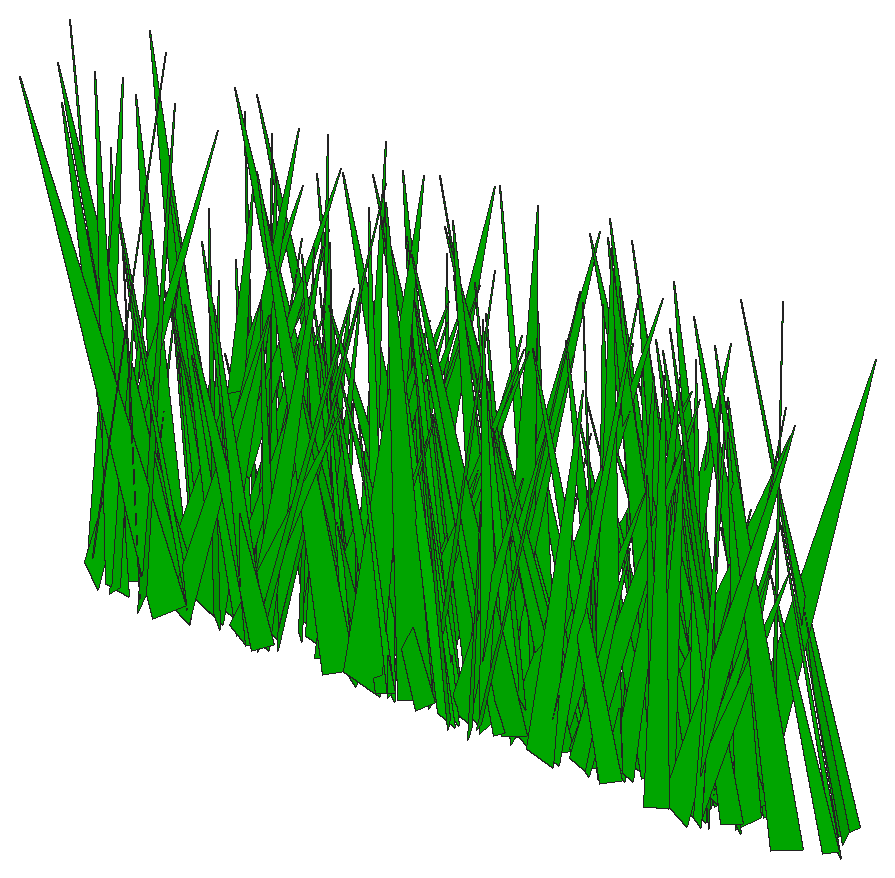
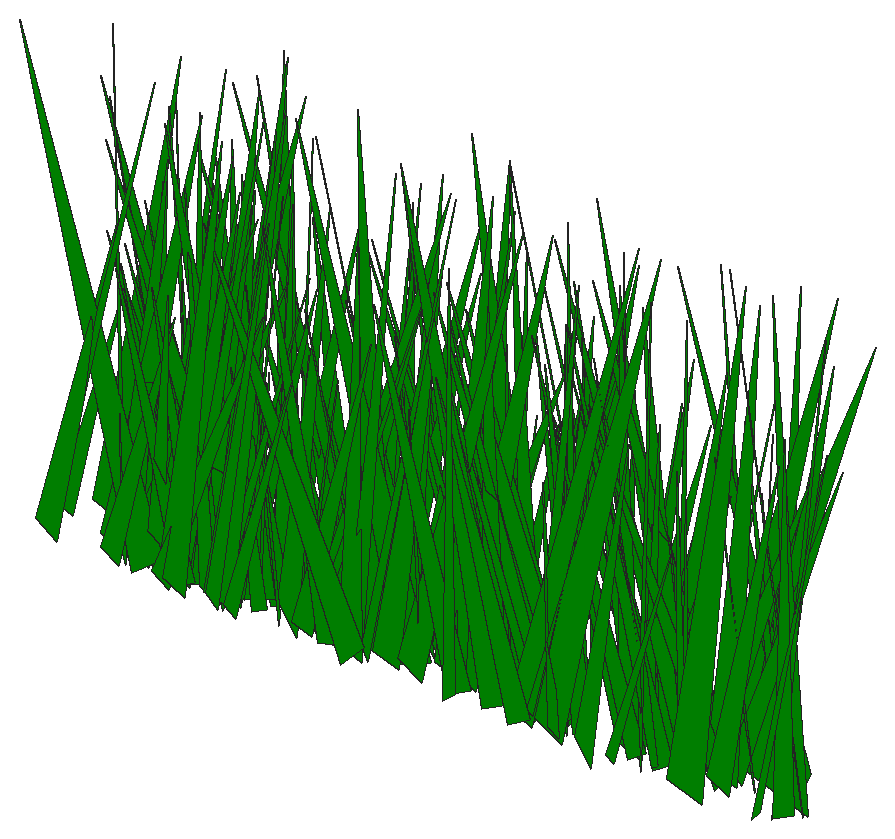
# SketchUp Ruby script. Lengths in inches.
U = 1.inch
M = Sketchup.active_model
def pt(a) = Geom::Point3d.new(a.map { |v| v * U })
def face(e, loops, mat)
  f = e.add_face(loops[0].map { |a| pt(a) })
  loops[1..].each { |l| e.add_face(l.map { |a| pt(a) }).erase! }
  f.material = f.back_material = mat if mat
  f
end
# faces: each face lists its corners as indices into pts; further lists are holes
def faces(e, pts, list, mat = nil) = list.each { |f| face(e, (f[0].is_a?(Array) ? f : [f]).map { |l| l.map { |i| pts[i] } }, mat) }
# xy, xz, yz: faces in a plane at the given z, y or x. An outline is a flat list of corners, or four numbers for a rectangle; further outlines are holes
def ring(l) = l.size == 4 ? [[l[0], l[1]], [l[2], l[1]], [l[2], l[3]], [l[0], l[3]]] : l.each_slice(2).to_a
def flat(e, list, mat, &to3) = list.each { |f| face(e, (f[0].is_a?(Array) ? f : [f]).map { |l| ring(l).map { |u, v| to3.(u, v) } }, mat) }
def xy(e, z, list, mat = nil) = flat(e, list, mat) { |x, y| [x, y, z] }
def xz(e, y, list, mat = nil) = flat(e, list, mat) { |x, z| [x, y, z] }
def yz(e, x, list, mat = nil) = flat(e, list, mat) { |y, z| [x, y, z] }
def lines(e, pts, list) = list.each { |a, b| e.add_line(pt(pts[a]), pt(pts[b])) }
# prism: a flat outline (further loops are holes) pulled along v
def prism(e, loops, v, mat = nil)
  f = face(e, loops, mat); d = Geom::Vector3d.new(v.map { |x| x * U })
  f.pushpull(f.normal.samedirection?(d) ? d.length : -d.length)
end
def box(e, o, s, mat = nil) = prism(e, [[o, [o[0] + s[0], o[1], o[2]], [o[0] + s[0], o[1] + s[1], o[2]], [o[0], o[1] + s[1], o[2]]]], [0, 0, s[2]], mat)
def at(x, y, z, deg = 0) = Geom::Transformation.translation(pt([x, y, z])) * Geom::Transformation.rotation(ORIGIN, Z_AXIS, deg.degrees)
def axes(o, x, y, z) = Geom::Transformation.new([*x, 0, *y, 0, *z, 0, *pt(o).to_a, 1])
def part(name) = M.definitions.add(name)
# library, detail: a bought-in or finely detailed component or shape, given as its bounding box
def library(name, o, s) = part(name).tap { |d| box(d.entities, o, s) }
def detail(e, o, s) = box(e.add_group.entities, o, s)
def put(e, d, t, mat = nil) = e.add_instance(d, t).tap { |i| i.material = mat if mat }
def group(e, t, mat = nil) = e.add_group.tap { |g| g.transformation = t; g.material = mat if mat }.entities
root = M.entities
M.materials.add("[Color G06]").color = [0, 204, 0]
c1 = part("fur_instance\#9")
p = [[0.8125,0,1.79],[0.67,-0.02,1.48],[0,-0.11,0],[0,0.11,0]]
faces(c1.entities,p,[[0,1,2,3]])
put(root,c1,axes([35.12,20.5,4.28],[3.03106,0.62127,0.65652],[4.35449,-0.39194,-2.30003],[1.03981,-0.16965,7.71826]),"[Color G06]")
put(root,c1,axes([19.64,20.68,4.28],[-0.16092,-0.52107,1.62952],[-3.59911,-0.03804,-2.19139],[-1.48269,0.1489,5.14257]),"[Color G06]")
put(root,c1,axes([19.41,20.69,4.28],[0.64346,-0.50098,1.74087],[-3.60806,-0.13024,-1.32649],[-1.11623,0.13218,5.29122]),"[Color G06]")
put(root,c1,axes([35.98,20.48,4.28],[-4.26408,0.16313,3.37539],[0.76507,0.66856,-1.55286],[2.42564,0.0759,6.42343]),"[Color G06]")
put(root,c1,axes([16.83,20.84,4.28],[-4.57704,-0.06266,0.97472],[-0.21793,0.61243,2.2369],[0.76142,-0.20138,6.49945]),"[Color G06]")
put(root,c1,axes([19.34,20.78,4.28],[4.92761,0.10985,0.51711],[0.85255,-0.66121,-2.01124],[-0.11605,-0.19308,7.18189]),"[Color G06]")
put(root,c1,axes([34.49,20.44,4.28],[2.21235,0.64995,0.69926],[4.55515,-0.31532,1.47593],[-1.0927,0.00144,7.56847]),"[Color G06]")
put(root,c1,axes([35.93,21.02,4.28],[-4.71268,-0.24632,3.19454],[-0.77772,0.68157,3.47433],[2.6616,-0.23699,6.67152]),"[Color G06]")
put(root,c1,axes([26.68,20.53,4.28],[-4.24437,-0.06717,1.88959],[-0.90731,0.57193,-2.21683],[1.00363,0.23297,5.987]),"[Color G06]")
put(root,c1,axes([25.04,21.02,4.28],[1.87576,-0.80358,0.85838],[-5.66872,-0.272,-1.58046],[-1.18508,0.02914,8.91863]),"[Color G06]")
put(root,c1,axes([39.03,20.82,4.28],[0.00921,-0.7447,2.68248],[-5.44964,-0.06467,-2.02075],[-1.42936,0.24178,7.72166]),"[Color G06]")
put(root,c1,axes([27.5,20.5,4.28],[2.69023,0.2021,0.81048],[0.96941,-0.33831,2.5036],[-1.2062,0.17886,3.81975]),"[Color G06]")
put(root,c1,axes([19.36,20.75,4.28],[-2.87953,-0.43874,1.8429],[-3.37542,0.38429,-1.27127],[0.16259,0.20765,6.24647]),"[Color G06]")
put(root,c1,axes([30.03,20.59,4.28],[-0.85297,0.60878,1.16187],[4.29251,0.14106,-1.45105],[1.11278,-0.07747,6.48798]),"[Color G06]")
put(root,c1,axes([24.27,20.86,4.28],[-2.92029,0.05795,1.28824],[0.62873,0.40718,1.07968],[0.72134,-0.12032,4.2743]),"[Color G06]")
put(root,c1,axes([35.49,20.8,4.28],[2.18325,-0.4105,0.47109],[-2.76341,-0.26295,2.28609],[1.06249,0.15961,4.97782]),"[Color G06]")
put(root,c1,axes([15.07,20.6875,4.28],[-3.72344,0.00901,1.8687],[-0.1721,0.53817,-1.06414],[1.24011,0.10175,5.46312]),"[Color G06]")
put(root,c1,axes([16.21,20.62,4.28],[-2.3339,0.80888,0.33748],[5.3635,0.28748,3.69996],[-2.22077,-0.15576,8.58131]),"[Color G06]")
put(root,c1,axes([18.57,20.84,4.28],[2.41753,-0.38371,0.07703],[-2.51991,-0.30476,2.26301],[1.10665,0.14429,4.98474]),"[Color G06]")
put(root,c1,axes([30.38,20.73,4.28],[5.62136,-0.17826,1.62606],[-1.45971,-0.78092,1.43755],[-0.82896,0.16627,8.49527]),"[Color G06]")
put(root,c1,axes([14.17,20.625,4.28],[2.74687,0.29235,0.65447],[1.88385,-0.37704,1.68599],[-1.01892,0.09103,4.88158]),"[Color G06]")
put(root,c1,axes([32.51,20.79,4.28],[-3.33536,0.46956,1.16031],[3.453,0.44692,1.39501],[-0.13635,-0.16822,6.94495]),"[Color G06]")
put(root,c1,axes([35.52,20.76,4.28],[3.05836,-0.22556,0.72653],[-1.67747,-0.38928,1.88997],[0.19704,0.18691,4.8131]),"[Color G06]")
put(root,c1,axes([34.02,21.12,4.28],[-2.60033,-0.46267,0.25722],[-3.10158,0.34898,2.06931],[1.19093,-0.10135,5.9508]),"[Color G06]")
put(root,c1,axes([16.48,20.74,4.28],[2.02147,0.50228,0.40268],[3.50973,-0.26296,-1.67687],[0.8536,-0.10826,5.94115]),"[Color G06]")
put(root,c1,axes([34.1,21.12,4.28],[-0.32855,-0.64108,0.01669],[-4.51737,0.04531,1.27825],[0.85387,-0.00698,6.76896]),"[Color G06]")
put(root,c1,axes([27.64,21.27,4.28],[4.3846,-0.48787,0.56481],[-3.03521,-0.56691,-3.62029],[-1.78067,-0.23498,7.56167]),"[Color G06]")
put(root,c1,axes([14.2,20.71,4.28],[-4.583,0.48117,1.87027],[3.37343,0.66218,-1.10489],[1.44648,-0.01979,8.50251]),"[Color G06]")
put(root,c1,axes([22.67,20.93,4.28],[2.25118,0.34416,0.97871],[2.47695,-0.26475,-2.03182],[0.62042,-0.19181,4.56054]),"[Color G06]")
put(root,c1,axes([36.72,21.24,4.28],[-5.18037,-0.44074,0.71566],[-2.90398,0.70198,2.70695],[1.3364,-0.18308,8.65635]),"[Color G06]")
put(root,c1,axes([15.23,20.54,4.28],[5.5582,0.36566,1.922],[1.96819,-0.75378,3.76014],[-2.15785,0.25435,8.38033]),"[Color G06]")
put(root,c1,axes([17.59,21.1,4.28],[4.26432,0.09876,3.43905],[1.41152,-0.63127,-1.82705],[-1.95037,-0.24093,6.19693]),"[Color G06]")
put(root,c1,axes([26.49,20.67,4.28],[-5.24823,0.34183,0.47936],[2.34477,0.72151,-1.75957],[0.78352,0.13044,8.47659]),"[Color G06]")
put(root,c1,axes([24.1,20.8,4.28],[-0.67427,0.46476,0.38897],[3.23485,0.08136,1.35845],[-0.84375,-0.05948,4.89731]),"[Color G06]")
put(root,c1,axes([34.95,21.02,4.28],[3.93696,0.08139,0.63429],[0.66802,-0.53518,-1.37349],[-0.27293,-0.13593,5.78765]),"[Color G06]")
put(root,c1,axes([36.79,21.06,4.28],[-0.11601,-0.52436,1.11552],[-3.72432,-0.00928,-1.36638],[-0.90927,0.10492,5.45426]),"[Color G06]")
put(root,c1,axes([23.22,20.79,4.28],[-0.49886,0.82731,2.40594],[5.98908,0.11619,-1.81578],[1.38616,-0.20428,8.71119]),"[Color G06]")
put(root,c1,axes([25.5,20.92,4.28],[-0.30634,0.47925,1.93309],[3.28373,-0.04526,2.45133],[-1.64365,-0.17974,4.53704]),"[Color G06]")
put(root,c1,axes([31.09,20.98,4.28],[1.57776,-0.32972,0.79265],[-2.38807,-0.19659,1.22427],[0.41125,0.1234,4.06817]),"[Color G06]")
put(root,c1,axes([37.18,21.34,4.28],[3.35801,-0.57328,0.19361],[-3.78603,-0.43991,-2.9546],[-1.60756,-0.16146,7.3629]),"[Color G06]")
put(root,c1,axes([19.23,20.91,4.28],[2.25077,0.58808,1.62519],[4.34639,-0.29243,-1.29023],[0.27748,-0.1897,7.0271]),"[Color G06]")
put(root,c1,axes([28.6,21.31,4.28],[4.65218,-0.31999,3.02467],[-1.4148,-0.68035,-3.4076],[-2.71291,-0.19393,6.96387]),"[Color G06]")
put(root,c1,axes([15.91,21.14,4.28],[-1.41791,-0.8139,1.79723],[-5.73201,0.13912,-2.86391],[-1.62996,0.21876,8.50796]),"[Color G06]")
put(root,c1,axes([32.02,20.88,4.28],[-4.91073,-0.09175,2.93937],[-1.09973,0.71287,-1.54788],[1.75824,0.18962,7.24145]),"[Color G06]")
put(root,c1,axes([26.59,21.13,4.28],[1.04517,-0.44785,0.3848],[-3.08103,-0.12788,1.59541],[0.94243,0.07859,4.78905]),"[Color G06]")
put(root,c1,axes([25.52,21.18,4.28],[5.42184,-0.07885,1.38292],[-0.3993,-0.75684,-1.4605],[-1.00821,-0.1243,8.01532]),"[Color G06]")
put(root,c1,axes([36.54,21.33,4.28],[-3.5413,-0.41182,0.07637],[-2.82796,0.47593,1.90196],[0.85281,-0.1319,6.62408]),"[Color G06]")
put(root,c1,axes([28.61,21.16,4.28],[-2.8689,-0.64055,0.93156],[-4.58066,0.37601,-1.80997],[-0.71213,0.1619,7.88945]),"[Color G06]")
put(root,c1,axes([19.78,21.1875,4.28],[6.16936,0.07955,0.8439],[0.67537,-0.84425,-1.88696],[-0.43372,-0.18313,9.0656]),"[Color G06]")
put(root,c1,axes([35.68,20.85,4.28],[-4.41516,0.36248,1.9516],[2.30711,0.63792,-1.95194],[1.77187,0.07262,7.40458]),"[Color G06]")
put(root,c1,axes([22.27,20.93,4.28],[-0.35866,0.7597,1.88035],[5.33757,-0.00585,2.54559],[-1.66556,-0.18234,7.75287]),"[Color G06]")
put(root,c1,axes([18.78,20.95,4.28],[-1.105,0.42188,0.11857],[2.93685,0.14663,1.20482],[-0.73109,-0.04864,4.66069]),"[Color G06]")
put(root,c1,axes([31.06,21.12,4.28],[3.73719,0.49583,1.01531],[3.52225,-0.46662,-2.78296],[0.8356,-0.25063,7.18986]),"[Color G06]")
put(root,c1,axes([27.48,20.93,4.28],[5.57106,0.18803,0.56765],[1.26489,-0.76851,1.51381],[-0.60214,0.12531,8.43197]),"[Color G06]")
put(root,c1,axes([31.92,21.33,4.28],[3.69445,-0.67086,2.00041],[-4.7944,-0.54145,-1.08036],[-1.3965,0.0841,9.00119]),"[Color G06]")
put(root,c1,axes([22.82,21.14,4.28],[2.54448,0.33779,0.70213],[2.43032,-0.32681,-1.61237],[0.42666,-0.15291,4.99697]),"[Color G06]")
put(root,c1,axes([26.54,21.26,4.28],[-2.97565,0.01103,1.03454],[0.27155,0.40828,1.24463],[0.6416,-0.12164,4.27124]),"[Color G06]")
put(root,c1,axes([13.81,21.05,4.28],[3.82908,-0.09459,2.02127],[-1.05218,-0.53525,1.57494],[-1.08723,0.18486,5.59449]),"[Color G06]")
put(root,c1,axes([23.23,21.22,4.28],[-3.99076,-0.33553,0.30649],[-2.39896,0.54449,-1.29951],[-0.27685,0.11844,6.84243]),"[Color G06]")
put(root,c1,axes([22.52,21.08,4.28],[-4.08598,0.15524,1.44869],[0.93993,0.58036,-1.22225],[1.13814,0.07801,6.21026]),"[Color G06]")
put(root,c1,axes([13.06,20.93,4.28],[5.98017,-0.1921,1.59286],[-1.71071,-0.74768,3.98827],[-0.32724,0.39808,8.25937]),"[Color G06]")
put(root,c1,axes([28.31,21.19,4.28],[-2.50155,0.55606,1.41368],[4.01936,0.30269,2.21007],[-0.80048,-0.21785,6.67933]),"[Color G06]")
put(root,c1,axes([30.36,21.33,4.28],[-1.19018,-0.46633,1.20952],[-3.31811,0.12397,-1.80256],[-0.91021,0.15783,4.98957]),"[Color G06]")
put(root,c1,axes([28.74,21.23,4.28],[4.54535,0.58511,0.37353],[4.11692,-0.60933,-2.25946],[0.8482,-0.17795,8.96505]),"[Color G06]")
put(root,c1,axes([24.04,21.02,4.28],[-3.86115,0.3343,0.70905],[1.95591,0.49689,-3.12007],[1.46517,0.21766,6.03365]),"[Color G06]")
put(root,c1,axes([29.82,21.36,4.28],[1.90983,-0.43639,1.0195],[-3.01462,-0.20749,2.41207],[1.0822,0.19215,4.91998]),"[Color G06]")
put(root,c1,axes([19.29,21.52,4.28],[-2.70255,-0.39023,1.22922],[-2.68009,0.39392,1.20348],[1.15099,0.00098,5.68854]),"[Color G06]")
put(root,c1,axes([34.15,21.53,4.28],[0.15749,-0.83898,2.44528],[-6.10794,-0.06661,-1.74668],[-1.25267,0.21931,8.8241]),"[Color G06]")
put(root,c1,axes([26.29,21.02,4.28],[-4.98773,0.42535,0.0635],[2.86559,0.65716,-2.89905],[1.04623,0.22784,8.24313]),"[Color G06]")
put(root,c1,axes([17.09,21.39,4.28],[3.61493,0.65317,2.23782],[4.91376,-0.46964,-1.98394],[0.19252,-0.27773,8.61759]),"[Color G06]")
put(root,c1,axes([21.77,21.54,4.28],[0.60564,-0.61854,1.69679],[-4.48522,-0.11225,-1.12457],[-0.92052,0.13998,6.59585]),"[Color G06]")
put(root,c1,axes([32.4375,21.44,4.28],[-0.85714,-0.47006,2.60488],[-3.49577,0.19476,1.46779],[1.47663,0.18821,4.9869]),"[Color G06]")
put(root,c1,axes([21.35,21.26,4.28],[3.67043,0.36059,1.03527],[2.49178,-0.5201,1.07645],[-0.97865,0.02816,6.62356]),"[Color G06]")
put(root,c1,axes([28.75,21.28,4.28],[-3.60971,-0.32931,2.99245],[-2.99666,0.47943,-2.01377],[0.77841,0.31855,6.1244]),"[Color G06]")
put(root,c1,axes([26.88,21.32,4.28],[3.19451,-0.29495,1.75851],[-2.41955,-0.38204,2.45717],[0.06335,0.28178,5.17213]),"[Color G06]")
put(root,c1,axes([33.71,21.32,4.28],[-2.17781,0.39947,0.93712],[2.65887,0.31492,-1.61868],[1.23705,0.0264,5.12894]),"[Color G06]")
put(root,c1,axes([14.27,21.46,4.28],[-1.80547,0.67445,1.82053],[4.92501,0.21252,1.86578],[-0.78831,-0.21696,7.48701]),"[Color G06]")
put(root,c1,axes([32.05,21.29,4.28],[2.70727,0.65205,1.32114],[4.48259,-0.39703,1.99169],[-1.59782,-0.00903,7.82601]),"[Color G06]")
put(root,c1,axes([24.07,21.53,4.28],[4.2436,-0.35839,0.16927],[-2.46631,-0.55809,2.37543],[0.7318,0.19737,7.02409]),"[Color G06]")
put(root,c1,axes([26.62,21.39,4.28],[3.30744,0.24109,0.79704],[1.54588,-0.45707,1.55276],[-0.94012,0.09661,5.35736]),"[Color G06]")
put(root,c1,axes([23.5,21.45,4.28],[2.60414,0.1253,1.1158],[0.66224,-0.36787,1.29287],[-0.96237,0.0859,3.90899]),"[Color G06]")
put(root,c1,axes([40.125,21.51,4.28],[-1.7987,0.35882,0.18815],[2.52485,0.24126,1.06131],[-0.51223,-0.07079,4.57067]),"[Color G06]")
put(root,c1,axes([23.78,21.84,4.28],[5.07038,0.2388,0.6504],[1.69099,-0.60234,-4.04173],[0.5124,-0.37521,6.90232]),"[Color G06]")
put(root,c1,axes([35.47,21.77,4.28],[5.18688,0.03411,1.13883],[0.44504,-0.70208,-2.11198],[-0.66512,-0.20376,7.46789]),"[Color G06]")
put(root,c1,axes([35.07,21.61,4.28],[0.23409,0.45872,2.43222],[3.38187,-0.1153,1.77092],[-1.42577,-0.19816,4.59988]),"[Color G06]")
put(root,c1,axes([15.09,21.63,4.28],[-3.24987,-0.41215,0.45613],[-2.87294,0.41976,-2.15305],[-0.75829,0.17602,6.20239]),"[Color G06]")
put(root,c1,axes([16.12,21.63,4.28],[-1.97766,0.50406,1.12542],[3.46058,0.2115,2.70201],[-1.28752,-0.20578,5.53376]),"[Color G06]")
put(root,c1,axes([27.38,21.78,4.28],[2.40972,-0.65697,2.77663],[-4.71727,-0.39556,-1.60647],[-1.84257,0.1535,7.7441]),"[Color G06]")
put(root,c1,axes([26.76,21.87,4.28],[0.27251,-0.5049,0.06103],[-3.50501,-0.03821,-1.3579],[-0.90901,-0.00401,5.25414]),"[Color G06]")
put(root,c1,axes([17.48,21.7,4.28],[3.79399,-0.27301,0.18763],[-1.93574,-0.51476,1.3933],[0.31881,0.12341,6.22688]),"[Color G06]")
put(root,c1,axes([32.19,21.39,4.28],[-4.10626,0.43516,0.58348],[2.85415,0.55323,-2.53012],[1.32084,0.15737,7.28118]),"[Color G06]")
put(root,c1,axes([30.22,21.74,4.28],[-3.29677,-0.6573,1.53149],[-4.70067,0.39892,-2.93517],[-1.08265,0.26948,8.08042]),"[Color G06]")
put(root,c1,axes([23.38,21.42,4.28],[-4.88738,0.35685,1.49787],[2.1409,0.67312,-2.81805],[1.72335,0.17582,7.74879]),"[Color G06]")
put(root,c1,axes([31.58,21.53,4.28],[-2.66533,0.26974,0.25786],[1.80189,0.35872,-1.50297],[0.72445,0.10019,4.687]),"[Color G06]")
put(root,c1,axes([19.29,21.41,4.28],[5.38754,0.19095,3.5059],[0.36145,-0.77054,3.58038],[-2.69204,0.27869,7.49702]),"[Color G06]")
put(root,c1,axes([32.375,21.96,4.28],[-0.98444,-0.64933,1.24012],[-4.60765,0.15835,1.35416],[1.06832,0.0846,6.98327]),"[Color G06]")
put(root,c1,axes([16.68,21.6,4.28],[-1.52174,0.33683,0.27529],[2.20042,0.20488,-1.62616],[1.01327,0.06095,3.9448]),"[Color G06]")
put(root,c1,axes([25.5625,21.78,4.28],[-0.67103,0.57299,2.52442],[3.89391,-0.03882,3.3244],[-2.13888,-0.25045,5.26021]),"[Color G06]")
put(root,c1,axes([17.5625,21.75,4.28],[-1.88148,0.58726,1.76168],[4.34734,0.2317,1.49858],[-0.47559,-0.20535,6.72902]),"[Color G06]")
put(root,c1,axes([35.65,21.75,4.28],[2.24277,-0.31165,1.59448],[-2.47175,-0.2693,1.71954],[0.15293,0.21775,4.40863]),"[Color G06]")
put(root,c1,axes([33.28,21.77,4.28],[-2.21003,0.46612,0.66655],[3.31705,0.28707,1.50624],[-0.60781,-0.12819,5.79654]),"[Color G06]")
put(root,c1,axes([33.21,21.85,4.28],[1.96878,0.63767,2.01723],[4.34383,-0.15593,-3.80749],[1.96579,-0.29407,6.39314]),"[Color G06]")
put(root,c1,axes([12.36,22.1,4.28],[4.87288,-0.42927,1.62301],[-2.9059,-0.69439,-1.60957],[-1.48722,-0.04974,8.46277]),"[Color G06]")
put(root,c1,axes([15.28,22.02,4.28],[2.16634,-0.67824,2.53769],[-4.87924,-0.35255,-1.51985],[-1.65314,0.15175,7.81131]),"[Color G06]")
put(root,c1,axes([32.36,22.14,4.28],[-0.23066,-0.71514,0.54641],[-4.99104,0.0434,1.81849],[1.23454,0.04184,7.45396]),"[Color G06]")
put(root,c1,axes([40.23,21.6875,4.28],[-3.79499,0.10997,0.12265],[0.71153,0.49705,-2.0156],[0.34977,0.18198,5.43109]),"[Color G06]")
put(root,c1,axes([31.61,22.06,4.28],[1.30861,-0.49054,0.09105],[-3.45578,-0.17751,1.08591],[0.66023,0.04314,5.50344]),"[Color G06]")
put(root,c1,axes([14.41,21.63,4.28],[3.90257,0.21687,0.92757],[1.13038,-0.50313,2.88964],[-1.23536,0.22473,5.5743]),"[Color G06]")
put(root,c1,axes([22.42,21.83,4.28],[4.88543,-0.34726,3.68876],[-3.00301,-0.7191,1.10746],[-1.80971,0.25582,8.12036]),"[Color G06]")
put(root,c1,axes([15.49,21.78,4.28],[3.06956,0.66655,0.29466],[4.64934,-0.40793,-2.18422],[1.12751,-0.13254,8.20453]),"[Color G06]")
put(root,c1,axes([16.82,22.16,4.28],[-0.65445,-0.71745,1.06277],[-5.05125,0.11118,1.67399],[1.20909,0.07615,7.56868]),"[Color G06]")
put(root,c1,axes([33.54,21.9,4.28],[1.06131,0.6918,2.98216],[5.15125,-0.20838,1.45808],[-1.43475,-0.23642,7.44099]),"[Color G06]")
put(root,c1,axes([20.97,22.06,4.28],[2.40354,-0.54687,0.7576],[-3.80213,-0.29687,2.32758],[1.08662,0.17087,6.46853]),"[Color G06]")
put(root,c1,axes([34.94,22.1,4.28],[-1.92945,-0.80746,2.07379],[-5.78095,0.20528,-2.83256],[-1.42697,0.26017,8.67126]),"[Color G06]")
put(root,c1,axes([18.04,21.9375,4.28],[-3.64827,-0.09407,0.10951],[-0.66618,0.48593,-1.62579],[-0.12894,0.15096,5.30133]),"[Color G06]")
put(root,c1,axes([20.07,21.88,4.28],[4.22734,0.07162,2.54376],[0.04641,-0.61646,1.82159],[-1.7772,0.15426,6.09828]),"[Color G06]")
put(root,c1,axes([34.22,22.28,4.28],[0.69181,-0.81514,1.35676],[-5.79761,-0.11876,-1.59313],[-1.17599,0.10596,8.65221]),"[Color G06]")
put(root,c1,axes([20.75,21.85,4.28],[-2.53669,0.54539,1.23702],[3.80918,0.37123,-1.35322],[1.21332,-0.02521,6.83462]),"[Color G06]")
put(root,c1,axes([35.81,21.99,4.28],[-2.25849,0.52052,0.42224],[3.44366,0.27085,2.78917],[-1.46784,-0.16546,5.89393]),"[Color G06]")
put(root,c1,axes([28.46,21.89,4.28],[3.80868,0.09483,0.50705],[0.55462,-0.51212,1.6963],[-0.51954,0.14845,5.52797]),"[Color G06]")
put(root,c1,axes([22.54,22.01,4.28],[-3.11898,-0.31708,1.51864],[-2.48275,0.41379,-1.46537],[0.19687,0.19497,5.57959]),"[Color G06]")
put(root,c1,axes([27.11,22.15,4.28],[4.02419,0.3082,1.35497],[2.38606,-0.53057,-1.96604],[-0.11584,-0.22219,6.57417]),"[Color G06]")
put(root,c1,axes([30.99,22.57,4.28],[4.47502,-0.52241,0.82716],[-2.86354,-0.54497,-4.93304],[-2.47822,-0.31364,7.19366]),"[Color G06]")
put(root,c1,axes([24.93,22.12,4.28],[0.83098,-0.70142,3.77584],[-5.14173,-0.2395,-2.58326],[-2.2906,0.28315,7.16846]),"[Color G06]")
put(root,c1,axes([20.88,22.2,4.28],[0.98742,-0.65953,1.97394],[-4.4406,-0.03973,3.43713],[2.09641,0.22649,6.35075]),"[Color G06]")
put(root,c1,axes([27.67,22.38,4.28],[-1.20214,-0.83931,1.55845],[-5.98364,0.19161,1.54417],[1.22901,0.11193,9.04246]),"[Color G06]")
put(root,c1,axes([28.35,21.99,4.28],[-2.51012,0.25921,0.7144],[1.67036,0.34907,-1.43982],[0.94541,0.07148,4.44068]),"[Color G06]")
put(root,c1,axes([16.27,22.1,4.28],[5.39494,-0.36473,0.63116],[-2.62307,-0.71648,2.52093],[0.37301,0.23682,8.59888]),"[Color G06]")
put(root,c1,axes([35.61,22.47,4.28],[1.23077,-0.72707,0.73721],[-4.95178,-0.18456,-2.44306],[-1.70555,0.01116,7.62503]),"[Color G06]")
put(root,c1,axes([25.3,22.11,4.28],[1.51884,0.71777,3.10548],[5.29537,-0.27745,1.58139],[-1.66475,-0.22767,7.86354]),"[Color G06]")
put(root,c1,axes([18.77,22.23,4.28],[3.9578,0.30775,0.78399],[2.26535,-0.52858,-1.71019],[0.1177,-0.17476,6.55322]),"[Color G06]")
put(root,c1,axes([18.13,21.92,4.28],[-3.6391,0.33992,0.46182],[2.18449,0.48282,-2.37262],[1.12494,0.16203,6.10125]),"[Color G06]")
put(root,c1,axes([18.3,22.47,4.28],[3.91528,-0.52124,1.108],[-3.57063,-0.55357,-1.73178],[-1.33139,-0.04823,7.90277]),"[Color G06]")
put(root,c1,axes([20.73,22.07,4.28],[-5.22277,0.17087,3.28956],[0.88449,0.78588,-1.55264],[2.35874,0.08366,7.86602]),"[Color G06]")
put(root,c1,axes([12.28,22,4.28],[5.99572,0.15622,1.79283],[0.84066,-0.8364,2.09222],[-1.40972,0.16566,8.8728]),"[Color G06]")
put(root,c1,axes([20.36,22.34,4.28],[3.97982,0.02249,2.44013],[0.54873,-0.58121,-1.38371],[-1.54612,-0.14838,5.78997]),"[Color G06]")
put(root,c1,axes([30.77,22.0625,4.28],[-3.12616,-0.02513,1.0636],[-0.46077,0.40511,-1.92543],[0.5715,0.18913,4.2656]),"[Color G06]")
put(root,c1,axes([15.96,22.375,4.28],[-2.68835,0.001,1.49008],[0.42685,0.36247,1.69239],[0.90103,-0.16875,3.64414]),"[Color G06]")
put(root,c1,axes([36.79,22.24,4.28],[-2.93216,-0.53392,0.95106],[-3.71231,0.3533,-2.78112],[-1.13325,0.22413,6.64968]),"[Color G06]")
put(root,c1,axes([21.59,22.14,4.28],[1.89179,0.62725,0.50493],[4.28372,-0.23381,-2.48528],[1.41336,-0.13094,6.85673]),"[Color G06]")
put(root,c1,axes([37.08,22.5,4.28],[0.17084,-0.6719,0.82413],[-4.78778,-0.03563,-1.12021],[-0.77323,0.07218,7.11832]),"[Color G06]")
put(root,c1,axes([32.91,22.03,4.28],[-0.06281,0.77927,0.64327],[5.39784,0.02457,-2.24244],[1.5094,-0.05545,8.04609]),"[Color G06]")
put(root,c1,axes([21.64,22.39,4.28],[-2.3096,0.19192,1.04636],[1.54317,0.28056,1.69709],[-0.05552,-0.18586,3.64234]),"[Color G06]")
put(root,c1,axes([37.57,22.31,4.28],[-1.51914,0.69109,2.83758],[5.1931,0.13677,2.38365],[-1.09448,-0.31026,7.3714]),"[Color G06]")
put(root,c1,axes([23.27,22.59,4.28],[-2.08283,-0.6716,0.73205],[-4.6422,0.29817,1.92108],[1.3734,-0.01068,7.6036]),"[Color G06]")
put(root,c1,axes([32.35,22.16,4.28],[-2.81584,0.0773,1.16112],[0.20815,0.37911,-1.77171],[0.93141,0.14897,3.90625]),"[Color G06]")
put(root,c1,axes([21.65,22.3,4.28],[3.02328,0.45392,0.8269],[3.2479,-0.39,-1.93241],[0.59448,-0.17773,6.35232]),"[Color G06]")
put(root,c1,axes([15.04,22.27,4.28],[3.78659,-0.34094,0.09637],[-2.23136,-0.47478,2.89378],[1.00146,0.23125,6.08333]),"[Color G06]")
put(root,c1,axes([20.625,22.58,4.28],[4.22235,-0.091,2.35328],[-0.04094,-0.59181,-2.46485],[-1.70394,-0.21128,5.89063]),"[Color G06]")
put(root,c1,axes([33.18,22.66,4.28],[1.62393,-0.67104,0.27673],[-4.69696,-0.22671,-1.58459],[-1.06313,-0.02338,7.42346]),"[Color G06]")
put(root,c1,axes([20.04,22.48,4.28],[-0.85306,-0.52299,2.07441],[-3.79863,0.16784,1.37161],[1.25029,0.1531,5.58255]),"[Color G06]")
put(root,c1,axes([37.02,22.65,4.28],[5.76167,-0.0974,3.07915],[-0.07644,-0.82189,-2.66701],[-2.17406,-0.22923,8.25411]),"[Color G06]")
put(root,c1,axes([29.91,22.6,4.28],[-4.77693,0.0442,0.11301],[0.32582,0.64484,1.79039],[-0.00628,-0.16738,6.92755]),"[Color G06]")
put(root,c1,axes([16.12,22.65,4.28],[-2.77613,-0.20322,1.50563],[-1.10455,0.4027,1.69472],[1.38518,-0.08617,4.36892]),"[Color G06]")
put(root,c1,axes([26.4375,22.32,4.28],[2.39113,0.79736,1.06186],[5.62473,-0.29972,-2.43819],[1.25049,-0.17652,8.93659]),"[Color G06]")
put(root,c1,axes([16.97,22.63,4.28],[0.39983,-0.49909,0.60828],[-3.35387,-0.03075,2.02647],[1.31422,0.07338,4.98647]),"[Color G06]")
put(root,c1,axes([33.97,22.25,4.28],[-2.32376,0.30542,0.29951],[1.86573,0.29526,-2.25336],[1.16471,0.1364,4.20717]),"[Color G06]")
put(root,c1,axes([17.51,22.38,4.28],[4.3873,0.13638,1.08087],[0.86214,-0.61493,1.09631],[-0.85806,0.07947,6.62803]),"[Color G06]")
put(root,c1,axes([36.13,22.64,4.28],[-0.36819,-0.80692,3.17032],[-5.42227,0.18327,3.95203],[2.92983,0.23778,7.71247]),"[Color G06]")
put(root,c1,axes([15.03,22.48,4.28],[0.00326,0.53434,2.18722],[3.88937,-0.06523,1.81769],[-1.30305,-0.19336,5.43095]),"[Color G06]")
put(root,c1,axes([31.15,22.73,4.28],[3.77337,0.02294,1.49058],[0.56545,-0.49341,-2.3251],[-0.83785,-0.22968,5.14384]),"[Color G06]")
put(root,c1,axes([34.71,22.36,4.28],[-3.47918,0.03032,1.0474],[-0.05782,0.46075,-1.96144],[0.73149,0.18065,4.82672]),"[Color G06]")
put(root,c1,axes([17.95,22.59,4.28],[2.3278,-0.39983,0.46104],[-2.79798,-0.29975,1.69468],[0.69833,0.13179,5.2532]),"[Color G06]")
put(root,c1,axes([33.78,22.78,4.28],[3.94855,-0.35011,0.92956],[-2.33441,-0.55051,-1.66868],[-1.11403,-0.08734,6.79138]),"[Color G06]")
put(root,c1,axes([32.76,22.43,4.28],[-4.80675,0.03612,1.82161],[0.0279,0.68026,-1.38517],[1.24573,0.12415,7.05987]),"[Color G06]")
put(root,c1,axes([33.24,22.86,4.28],[-4.61256,0.01157,0.94025],[0.38659,0.56168,3.44216],[0.5032,-0.32544,5.97424]),"[Color G06]")
put(root,c1,axes([17.08,22.61,4.28],[4.40817,-0.30173,0.57795],[-2.19784,-0.6069,1.04704],[-0.03393,0.11148,7.26419]),"[Color G06]")
put(root,c1,axes([21.73,22.48,4.28],[5.10989,-0.0953,0.07629],[-0.67614,-0.69228,1.81622],[0.11194,0.16888,7.488]),"[Color G06]")
put(root,c1,axes([39.77,22.79,4.28],[1.37065,-0.52504,1.35157],[-3.37435,-0.22757,-2.51145],[-1.89955,0.0254,5.43658]),"[Color G06]")
put(root,c1,axes([31.93,22.69,4.28],[-0.59305,-0.36167,1.00224],[-2.50797,0.10862,1.18792],[0.9417,0.06152,3.79486]),"[Color G06]")
put(root,c1,axes([34.31,22.51,4.28],[-0.44203,0.45339,1.22495],[3.17071,0.09402,-1.44193],[1.09088,-0.08956,4.6874]),"[Color G06]")
put(root,c1,axes([26.3125,22.7,4.28],[-3.66695,-0.62321,1.00797],[-4.47964,0.48501,-1.95468],[-0.60123,0.18729,8.41616]),"[Color G06]")
put(root,c1,axes([39.92,22.45,4.28],[-5.84389,-0.20268,1.24201],[-1.64477,0.77361,-2.78454],[0.31293,0.28111,8.55865]),"[Color G06]")
put(root,c1,axes([27.23,22.67,4.28],[1.41385,-0.55995,3.06638],[-4.14996,-0.27887,-1.57567],[-1.76403,0.20725,6.16448]),"[Color G06]")
put(root,c1,axes([16.35,22.5,4.28],[3.10974,-0.08097,2.58815],[-1.14148,-0.45838,1.41632],[-1.42582,0.19037,4.51094]),"[Color G06]")
put(root,c1,axes([21.63,22.625,4.28],[-4.29197,-0.33509,2.54453],[-2.75297,0.60555,-1.21188],[1.04602,0.2188,7.25106]),"[Color G06]")
put(root,c1,axes([35.18,22.51,4.28],[0.06624,0.70192,1.20227],[4.86587,-0.04214,2.2275],[-1.51928,-0.10437,7.18653]),"[Color G06]")
put(root,c1,axes([26.05,22.46,4.28],[-3.24261,0.11843,1.88617],[0.04823,0.42215,-2.85982],[1.52043,0.23919,4.11333]),"[Color G06]")
put(root,c1,axes([22.11,22.86,4.28],[-4.24902,-0.63239,0.73398],[-4.54084,0.57749,-1.56176],[-0.43393,0.1492,9.15584]),"[Color G06]")
put(root,c1,axes([28.31,22.99,4.28],[3.06301,-0.53057,0.99156],[-3.62375,-0.43564,-1.77335],[-1.33631,-0.0348,7.08171]),"[Color G06]")
put(root,c1,axes([37.37,22.875,4.28],[0.18734,-0.45054,0.81783],[-2.99624,-0.0545,-1.91582],[-1.32695,0.05945,4.44137]),"[Color G06]")
put(root,c1,axes([34.6,22.8125,4.28],[1.344,-0.45175,0.82324],[-3.16111,-0.15506,1.75312],[0.89782,0.13031,4.94017]),"[Color G06]")
put(root,c1,axes([21.15,22.9,4.28],[-0.06368,-0.83389,2.51979],[-5.78581,-0.07773,-3.28172],[-2.26452,0.22205,8.3139]),"[Color G06]")
put(root,c1,axes([34.75,22.52,4.28],[-5.75047,0.32814,0.51024],[2.24265,0.78987,-1.89502],[0.79024,0.14623,9.09084]),"[Color G06]")
put(root,c1,axes([20.77,22.97,4.28],[2.37895,-0.25566,0.30951],[-1.70404,-0.32251,-1.34589],[-0.70749,-0.08288,4.28238]),"[Color G06]")
put(root,c1,axes([12.81,22.53,4.28],[-5.90039,0.16754,1.65196],[0.83351,0.80614,-2.74156],[1.40372,0.22554,8.57178]),"[Color G06]")
put(root,c1,axes([22.97,22.76,4.28],[0.84669,0.78581,2.95747],[5.75065,-0.03199,-2.70116],[1.61311,-0.29842,8.07719]),"[Color G06]")
put(root,c1,axes([30.3,22.75,4.28],[-2.27248,0.43134,0.59747],[3.08308,0.30021,1.29599],[-0.47204,-0.11574,5.58831]),"[Color G06]")
put(root,c1,axes([27.95,22.76,4.28],[-5.66278,-0.19459,1.32907],[-1.53918,0.78173,-1.50098],[0.60747,0.16677,8.58643]),"[Color G06]")
put(root,c1,axes([35.88,22.6,4.28],[1.12455,0.49265,0.06447],[3.39368,-0.15237,1.52218],[-0.98314,0.03757,5.32813]),"[Color G06]")
put(root,c1,axes([16.06,22.66,4.28],[0.276,0.45763,0.04062],[3.11329,-0.03771,1.55434],[-1.03852,0.00857,4.67038]),"[Color G06]")
put(root,c1,axes([17.91,22.55,4.28],[5.11501,0.29007,3.35129],[1.02109,-0.73625,3.83924],[-2.88311,0.25386,7.30534]),"[Color G06]")
put(root,c1,axes([28.49,22.62,4.28],[-5.41799,0.39321,1.08225],[2.59371,0.74883,-2.24959],[1.32229,0.14231,8.84712]),"[Color G06]")
put(root,c1,axes([13.06,23.16,4.28],[-4.36412,-0.27076,0.34609],[-1.81767,0.59081,1.89884],[0.72101,-0.1494,6.88178]),"[Color G06]")
put(root,c1,axes([12.4,22.72,4.28],[-3.19187,0.46155,1.11568],[3.16054,0.45643,-1.49308],[1.23432,0.02483,6.70818]),"[Color G06]")
put(root,c1,axes([33.28,22.93,4.28],[-4.18697,0.55996,2.29718],[4.27323,0.57507,1.29495],[0.47643,-0.2369,8.57331]),"[Color G06]")
put(root,c1,axes([19.35,23.375,4.28],[3.2891,-0.45419,0.39747],[-2.51558,-0.38547,-4.10082],[-2.08604,-0.2513,5.57191]),"[Color G06]")
put(root,c1,axes([24.37,22.87,4.28],[0.83423,0.60259,1.07031],[4.19465,-0.08062,-2.08897],[1.2617,-0.1304,6.23732]),"[Color G06]")
put(root,c1,axes([21.92,23.13,4.28],[1.43894,-0.51335,0.3649],[-3.49705,-0.17813,2.017],[1.1758,0.09844,5.5524]),"[Color G06]")
put(root,c1,axes([24.42,23.25,4.28],[-3.90027,-0.39179,2.12018],[-2.45907,0.57592,2.12087],[1.96453,-0.05693,6.86405]),"[Color G06]")
put(root,c1,axes([29.13,22.96,4.28],[2.24918,0.56202,1.30447],[4.11426,-0.2964,-1.17632],[0.28037,-0.15915,6.79715]),"[Color G06]")
put(root,c1,axes([35.32,23.07,4.28],[-2.90693,0.37229,0.38623],[2.55405,0.36796,2.19587],[-0.81929,-0.17384,5.47496]),"[Color G06]")
put(root,c1,axes([28.16,23.09,4.28],[2.1463,0.62237,1.76279],[4.09915,-0.17352,-4.11103],[2.12316,-0.29414,6.15509]),"[Color G06]")
put(root,c1,axes([18.5,23.1875,4.28],[-2.5726,0.15727,0.35969],[1.15049,0.34437,1.08383],[-0.07929,-0.10597,4.05589]),"[Color G06]")
put(root,c1,axes([33.37,23.11,4.28],[-3.92163,-0.32245,1.85271],[-2.56717,0.53576,-1.42654],[0.54163,0.20467,6.65299]),"[Color G06]")
put(root,c1,axes([15.59,23.34,4.28],[1.4952,-0.79277,2.60513],[-5.66581,-0.26601,-2.03546],[-1.80507,0.17829,8.54685]),"[Color G06]")
put(root,c1,axes([32.58,23.26,4.28],[-2.49372,0.23896,0.94674],[1.82384,0.31686,1.54355],[-0.10688,-0.16829,4.25063]),"[Color G06]")
put(root,c1,axes([34.89,23.09,4.28],[1.63932,0.6894,2.70279],[4.9031,-0.2961,2.03321],[-1.91628,-0.16785,7.51444]),"[Color G06]")
